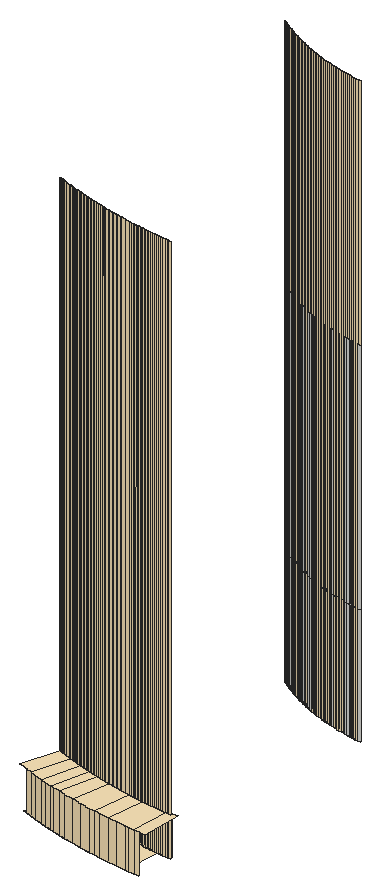
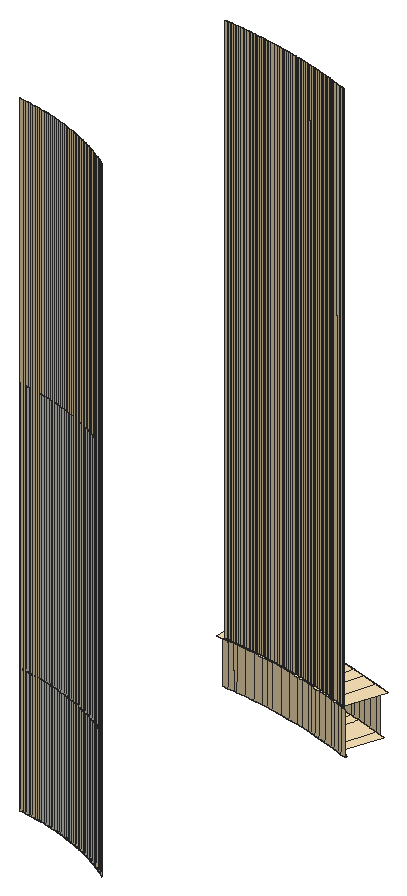
# SketchUp Ruby script. Lengths in inches.
U = 1.inch
M = Sketchup.active_model
def pt(a) = Geom::Point3d.new(a.map { |v| v * U })
def face(e, loops, mat)
  f = e.add_face(loops[0].map { |a| pt(a) })
  loops[1..].each { |l| e.add_face(l.map { |a| pt(a) }).erase! }
  f.material = f.back_material = mat if mat
  f
end
# faces: each face lists its corners as indices into pts; further lists are holes
def faces(e, pts, list, mat = nil) = list.each { |f| face(e, (f[0].is_a?(Array) ? f : [f]).map { |l| l.map { |i| pts[i] } }, mat) }
# xy, xz, yz: faces in a plane at the given z, y or x. An outline is a flat list of corners, or four numbers for a rectangle; further outlines are holes
def ring(l) = l.size == 4 ? [[l[0], l[1]], [l[2], l[1]], [l[2], l[3]], [l[0], l[3]]] : l.each_slice(2).to_a
def flat(e, list, mat, &to3) = list.each { |f| face(e, (f[0].is_a?(Array) ? f : [f]).map { |l| ring(l).map { |u, v| to3.(u, v) } }, mat) }
def xy(e, z, list, mat = nil) = flat(e, list, mat) { |x, y| [x, y, z] }
def xz(e, y, list, mat = nil) = flat(e, list, mat) { |x, z| [x, y, z] }
def yz(e, x, list, mat = nil) = flat(e, list, mat) { |y, z| [x, y, z] }
def lines(e, pts, list) = list.each { |a, b| e.add_line(pt(pts[a]), pt(pts[b])) }
# prism: a flat outline (further loops are holes) pulled along v
def prism(e, loops, v, mat = nil)
  f = face(e, loops, mat); d = Geom::Vector3d.new(v.map { |x| x * U })
  f.pushpull(f.normal.samedirection?(d) ? d.length : -d.length)
end
def box(e, o, s, mat = nil) = prism(e, [[o, [o[0] + s[0], o[1], o[2]], [o[0] + s[0], o[1] + s[1], o[2]], [o[0], o[1] + s[1], o[2]]]], [0, 0, s[2]], mat)
def at(x, y, z, deg = 0) = Geom::Transformation.translation(pt([x, y, z])) * Geom::Transformation.rotation(ORIGIN, Z_AXIS, deg.degrees)
def axes(o, x, y, z) = Geom::Transformation.new([*x, 0, *y, 0, *z, 0, *pt(o).to_a, 1])
def part(name) = M.definitions.add(name)
# library, detail: a bought-in or finely detailed component or shape, given as its bounding box
def library(name, o, s) = part(name).tap { |d| box(d.entities, o, s) }
def detail(e, o, s) = box(e.add_group.entities, o, s)
def put(e, d, t, mat = nil) = e.add_instance(d, t).tap { |i| i.material = mat if mat }
def group(e, t, mat = nil) = e.add_group.tap { |g| g.transformation = t; g.material = mat if mat }.entities
root = M.entities
M.materials.add("1026 AP 7946 SUNNY SIDE UP").color = [254, 231, 186]
xy(root,246,[[27.896,213.185,27.467,213.224,26.964,213.278,26.497,213.338,26.751,215.221,26.824,215.211,26.945,215.195,26.97,215.192,26.992,215.189,27.072,215.18,27.179,215.166,27.212,215.163,27.242,215.159,27.318,215.151,27.413,215.14,27.454,215.136,27.491,215.131,27.5625,215.124,27.648,215.116,27.697,215.111,27.741,215.107,27.806,215.101,27.882,215.094,27.94,215.089,27.992,215.084,28.05,215.08,28.055,215.079],[26.497,213.338,26.226,213.377,25.953,213.418,25.44,213.505,25.776,215.375,25.781,215.374,25.925,215.349,25.998,215.336,26.005,215.335,26.013,215.333,26.246,215.295,26.478,215.26,26.487,215.259,26.494,215.257,26.567,215.247,26.712,215.226,26.728,215.224,26.743,215.222,26.751,215.221],[25.44,213.505,24.926,213.603,24.465,213.699,24.87,215.555,24.94,215.54,25.01,215.524,25.047,215.517,25.087,215.508,25.181,215.489,25.256,215.473,25.286,215.468,25.318,215.461,25.424,215.441,25.503,215.425,25.525,215.421,25.549,215.416,25.67,215.394,25.75,215.379,25.765,215.377,25.776,215.375],[24.465,213.699,24.152,213.77,23.787,213.858,24.239,215.702,24.275,215.693,24.332,215.679,24.397,215.663,24.463,215.648,24.52,215.634,24.57,215.623,24.627,215.609,24.701,215.593,24.765,215.578,24.808,215.568,24.857,215.558,24.87,215.555],[23.787,213.858,23.573,213.912,23.274,213.99,23.768,215.823,23.788,215.818,23.857,215.8,23.94,215.778,23.988,215.765,24.031,215.754,24.095,215.738,24.168,215.719,24.225,215.705,24.239,215.702],
  [23.274,213.99,23.018,214.061,22.618,214.177,22.268,214.283,22.834,216.095,22.893,216.077,23.033,216.033,23.049,216.029,23.063,216.024,23.142,216.001,23.259,215.966,23.283,215.959,23.304,215.953,23.382,215.931,23.485,215.901,23.517,215.892,23.546,215.884,23.62,215.864,23.713,215.838,23.752,215.828,23.768,215.823],[22.268,214.283,22.016,214.364,21.774,214.444,22.379,216.242,22.584,216.175,22.808,216.103,22.816,216.101,22.823,216.098,22.834,216.095],[28.055,215.079,28.05,215.08,27.992,215.084,27.94,215.089,27.882,215.094,27.806,215.101,27.741,215.107,27.697,215.111,27.648,215.116,27.5625,215.124,27.491,215.131,27.454,215.136,27.413,215.14,27.318,215.151,27.242,215.159,27.212,215.163,27.179,215.166,27.072,215.18,26.992,215.189,26.97,215.192,26.945,215.195,26.824,215.211,26.751,215.221,26.764,215.32,27.198,215.265,27.664,215.214,28.064,215.178],[26.751,215.221,26.743,215.222,26.728,215.224,26.712,215.226,26.567,215.247,26.494,215.257,26.487,215.259,26.478,215.26,26.246,215.295,26.013,215.333,26.005,215.335,25.998,215.336,25.925,215.349,25.781,215.374,25.776,215.375,25.793,215.474,26.271,215.393,26.518,215.355,26.764,215.32],[25.776,215.375,25.765,215.377,25.75,215.379,25.67,215.394,25.549,215.416,25.525,215.421,25.503,215.425,25.424,215.441,25.318,215.461,25.286,215.468,25.256,215.473,25.181,215.489,25.087,215.508,25.047,215.517,25.01,215.524,24.94,215.54,24.87,215.555,24.891,215.653,25.317,215.564,25.793,215.474],
  [24.87,215.555,24.857,215.558,24.808,215.568,24.765,215.578,24.701,215.593,24.627,215.609,24.57,215.623,24.52,215.634,24.463,215.648,24.397,215.663,24.332,215.679,24.275,215.693,24.239,215.702,24.264,215.8,24.607,215.718,24.891,215.653],[24.239,215.702,24.225,215.705,24.168,215.719,24.095,215.738,24.031,215.754,23.988,215.765,23.94,215.778,23.857,215.8,23.788,215.818,23.768,215.823,23.794,215.922,24.072,215.848,24.264,215.8],[23.768,215.823,23.752,215.828,23.713,215.838,23.62,215.864,23.546,215.884,23.517,215.892,23.485,215.901,23.382,215.931,23.304,215.953,23.283,215.959,23.259,215.966,23.142,216.001,23.063,216.024,23.049,216.029,23.033,216.033,22.893,216.077,22.834,216.095,22.864,216.193,23.188,216.094,23.561,215.986,23.794,215.922],[22.834,216.095,22.823,216.098,22.816,216.101,22.808,216.103,22.584,216.175,22.379,216.242,22.411,216.34,22.634,216.266,22.864,216.193],[22.379,216.242,22.36,216.249,22.352,216.251,22.345,216.254,22.276,216.277,22.137,216.325,22.107,216.335,22.03,216.362,21.935,216.396,21.969,216.493,22.175,216.421,22.411,216.34]],"1026 AP 7946 SUNNY SIDE UP")
xy(root,248,[[28.983,213.12,29.064,215.118,28.752,215.132,28.503,215.147,28.378,213.151,28.649,213.135],[28.378,213.151,28.503,215.147,28.254,215.164,28.064,215.179,27.664,215.214,27.198,215.265,26.964,213.279,27.467,213.224,27.896,213.186,28.108,213.169],[26.964,213.279,27.198,215.265,26.765,215.32,26.518,215.355,26.226,213.377,26.497,213.338],[26.226,213.377,26.518,215.355,26.271,215.393,25.793,215.474,25.317,215.564,24.926,213.603,25.44,213.505,25.953,213.418],[24.926,213.603,25.317,215.564,24.891,215.653,24.607,215.718,24.152,213.77,24.465,213.699],
  [24.152,213.77,24.607,215.718,24.264,215.8,24.072,215.848,23.573,213.912,23.787,213.858],[23.573,213.912,24.072,215.848,23.794,215.922,23.561,215.986,23.018,214.061,23.274,213.99],[23.018,214.061,23.561,215.986,23.188,216.094,22.864,216.193,22.268,214.284,22.618,214.177],[22.268,214.284,22.864,216.193,22.634,216.266,22.412,216.34,22.175,216.421,21.519,214.531,21.774,214.444,22.016,214.364]],"1026 AP 7946 SUNNY SIDE UP")
p = [[28.649,213.135,246],[28.649,213.135,248],[28.378,213.151,248],[28.378,213.15,246],[27.467,213.224,246],[27.467,213.224,248],
  [26.964,213.279,248],[26.964,213.278,246],[27.896,213.185,246],[27.896,213.186,248],[28.108,213.169,246],[28.108,213.169,248],
  [26.497,213.338,246],[26.497,213.338,248],[26.226,213.377,248],[26.226,213.377,246],[25.953,213.418,246],[25.953,213.418,248],
  [25.44,213.505,248],[25.44,213.505,246],[24.926,213.603,248],[24.926,213.603,246],[24.465,213.699,248],[24.465,213.699,246],
  [24.152,213.77,248],[24.152,213.77,246],[23.787,213.858,248],[23.787,213.858,246],[23.573,213.912,246],[23.573,213.912,248],
  [23.274,213.99,248],[23.274,213.99,246],[23.018,214.061,248],[23.018,214.061,246],[22.618,214.177,248],[22.618,214.177,246],
  [22.268,214.284,248],[22.268,214.283,246],[22.016,214.364,248],[22.016,214.364,246],[28.428,215.052,246],[28.493,215.047,246],
  [28.493,215.047,274],[28.428,215.052,274],[28.538,215.045,246],[28.538,215.045,274],[28.587,215.042,246],[28.587,215.042,274],
  [28.673,215.037,246],[28.673,215.037,274],[28.744,215.033,246],[28.744,215.033,274],[27.318,215.151,246],[27.413,215.14,246],
  [27.413,215.14,274],[27.318,215.151,274],[27.454,215.136,246],[27.454,215.136,274],[27.491,215.131,246],[27.491,215.131,274],
  [27.5625,215.124,246],[27.5625,215.124,274],[27.648,215.116,246],[27.648,215.116,274],[27.697,215.111,246],[27.697,215.111,274],
  [27.741,215.107,246],[27.741,215.107,274],[27.806,215.101,246],[27.806,215.101,274],[27.882,215.094,246],[27.882,215.094,274],
  [27.94,215.089,246],[27.94,215.089,274],[27.992,215.084,246],[27.992,215.084,274],[28.05,215.08,246],[28.05,215.08,274],
  [28.055,215.079,246],[28.117,215.074,246],[28.117,215.074,274],[28.184,215.069,246],[28.184,215.069,274],[28.242,215.064,246],
  [28.242,215.064,274],[28.294,215.061,246],[28.294,215.061,274],[28.352,215.057,246],[28.352,215.057,274],[28.503,215.147,248],
  [28.503,215.146,246],[28.254,215.163,246],[28.254,215.164,248],[28.752,215.132,248],[28.752,215.132,246],[26.494,215.257,246],
  [26.567,215.247,246],[26.567,215.247,274],[26.494,215.257,274],[26.712,215.226,246],[26.712,215.226,274],[26.728,215.224,246],
  [26.728,215.224,274],[26.743,215.222,246],[26.743,215.222,274],[26.751,215.221,246],[26.824,215.211,246],[26.824,215.211,274],
  [26.945,215.195,246],[26.945,215.195,274],[26.97,215.192,246],[26.97,215.192,274],[26.992,215.189,246],[26.992,215.189,274],
  [27.072,215.18,246],[27.072,215.18,274],[27.179,215.166,246],[27.179,215.166,274],[27.212,215.163,246],[27.212,215.163,274],
  [27.242,215.159,246],[27.242,215.159,274],[27.664,215.214,248],[27.664,215.214,246],[27.198,215.265,246],[27.198,215.265,248],
  [28.064,215.179,248],[28.064,215.178,246],[25.781,215.374,246],[25.925,215.349,246],[25.925,215.349,274],[25.781,215.374,274],
  [25.998,215.336,246],[25.998,215.336,274],[26.005,215.335,246],[26.005,215.335,274],[26.013,215.333,246],[26.013,215.333,274],
  [26.246,215.295,246],[26.246,215.295,274],[26.478,215.26,246],[26.478,215.26,274],[26.487,215.259,246],[26.487,215.259,274],
  [26.765,215.32,248],[26.764,215.32,246],[26.518,215.355,246],[26.518,215.355,248],[25.318,215.461,246],[25.424,215.441,246],
  [25.424,215.441,274],[25.318,215.461,274],[25.503,215.425,246],[25.503,215.425,274],[25.525,215.421,246],[25.525,215.421,274],
  [25.549,215.416,246],[25.549,215.416,274],[25.67,215.394,246],[25.67,215.394,274],[25.75,215.379,246],[25.75,215.379,274],
  [25.765,215.377,246],[25.765,215.377,274],[25.776,215.375,246],[26.271,215.393,248],[26.271,215.393,246],[25.793,215.474,246],
  [25.793,215.474,248],[24.857,215.558,246],[24.87,215.555,246],[24.94,215.54,246],[24.94,215.54,274],[24.857,215.558,274],
  [25.01,215.524,246],[25.01,215.524,274],[25.047,215.517,246],[25.047,215.517,274],[25.087,215.508,246],[25.087,215.508,274],
  [25.181,215.489,246],[25.181,215.489,274],[25.256,215.473,246],[25.256,215.473,274],[25.286,215.468,246],[25.286,215.468,274],
  [25.317,215.564,246],[25.317,215.564,248],[24.397,215.663,246],[24.463,215.648,246],[24.463,215.648,274],[24.397,215.663,274],
  [24.52,215.634,246],[24.52,215.634,274],[24.57,215.623,246],[24.57,215.623,274],[24.627,215.609,246],[24.627,215.609,274],
  [24.701,215.593,246],[24.701,215.593,274],[24.765,215.578,246],[24.765,215.578,274],[24.808,215.568,246],[24.808,215.568,274],
  [24.891,215.653,246],[24.891,215.653,248],[24.031,215.754,246],[24.095,215.738,246],[24.095,215.738,274],[24.031,215.754,274],
  [24.168,215.719,246],[24.168,215.719,274],[24.225,215.705,246],[24.225,215.705,274],[24.239,215.702,246],[24.275,215.693,246],
  [24.275,215.693,274],[24.332,215.679,246],[24.332,215.679,274],[24.607,215.718,248],[24.607,215.718,246],[24.264,215.8,246],
  [24.264,215.8,248],[23.62,215.864,246],[23.713,215.838,246],[23.713,215.838,274],[23.62,215.864,274],[23.752,215.828,246],
  [23.752,215.828,274],[23.768,215.823,246],[23.788,215.818,246],[23.788,215.818,274],[23.857,215.8,246],[23.857,215.8,274],
  [24.072,215.848,248],[24.072,215.848,246],[23.794,215.922,246],[23.794,215.922,248],[23.94,215.778,246],[23.94,215.778,274],
  [23.988,215.765,246],[23.988,215.765,274],[23.304,215.953,246],[23.382,215.931,246],[23.382,215.931,274],[23.304,215.953,274],
  [23.485,215.901,246],[23.485,215.901,274],[23.517,215.892,246],[23.517,215.892,274],[23.546,215.884,246],[23.546,215.884,274],
  [23.561,215.986,246],[23.561,215.986,248],[22.893,216.077,246],[23.033,216.033,246],[23.033,216.033,274],[22.893,216.077,274],
  [23.049,216.029,246],[23.049,216.029,274],[23.063,216.024,246],[23.063,216.024,274],[23.142,216.001,246],[23.142,216.001,274],
  [23.259,215.966,246],[23.259,215.966,274],[23.188,216.094,246],[23.188,216.094,248],[23.283,215.959,246],[23.283,215.959,274],
  [22.584,216.175,246],[22.808,216.103,246],[22.808,216.103,274],[22.584,216.175,274],[22.816,216.101,246],[22.816,216.101,274],
  [22.823,216.098,246],[22.823,216.098,274],[22.834,216.095,246],[22.864,216.193,246],[22.864,216.193,248],[22.352,216.251,246],
  [22.36,216.249,246],[22.36,216.249,274],[22.352,216.251,274],[22.379,216.242,246],[22.634,216.266,246],[22.634,216.266,248],
  [22.107,216.335,246],[22.122,216.33,246],[22.122,216.33,274],[22.107,216.335,274],[22.137,216.325,246],[22.137,216.325,274],
  [22.276,216.277,246],[22.276,216.277,274],[22.412,216.34,248],[22.411,216.34,246],[22.175,216.421,246],[22.175,216.421,248],
  [22.345,216.254,246],[22.345,216.254,274],[21.969,216.493,246],[21.97,216.493,248],[28.123,227.148,252],[27.968,227.173,252],
  [27.968,227.173,246],[28.123,227.148,246],[28.123,227.148,246],[27.999,227.168,246],[27.999,227.168,276],[28.123,227.148,276],
  [28.278,227.124,252],[28.278,227.124,246],[28.247,227.129,246],[28.247,227.129,276],[28.371,227.111,246],[28.371,227.111,276],
  [28.434,227.103,252],[28.434,227.103,246],[28.59,227.083,252],[28.59,227.083,246],[28.496,227.095,246],[28.496,227.095,276],
  [28.621,227.08,246],[28.621,227.08,276],[28.746,227.066,252],[28.746,227.066,246],[28.746,227.066,246],[28.746,227.066,276],
  [27.659,227.231,252],[27.505,227.262,252],[27.505,227.262,246],[27.659,227.231,246],[27.628,227.237,246],[27.505,227.262,246],
  [27.505,227.262,276],[27.628,227.237,276],[27.751,227.213,246],[27.751,227.213,276],[27.813,227.201,252],[27.813,227.201,246],
  [27.875,227.19,246],[27.875,227.19,276],[27.199,227.332,252],[27.046,227.369,252],[27.046,227.369,246],[27.199,227.332,246],
  [27.138,227.346,246],[27.016,227.377,246],[27.016,227.377,276],[27.138,227.346,276],[27.26,227.317,246],[27.26,227.317,276],
  [27.352,227.296,252],[27.352,227.296,246],[27.382,227.289,246],[27.382,227.289,276],[26.894,227.409,252],[26.743,227.451,252],
  [26.743,227.451,246],[26.894,227.409,246],[26.773,227.442,246],[26.652,227.476,246],[26.652,227.476,276],[26.773,227.442,276],
  [26.894,227.409,246],[26.894,227.409,276],[26.442,227.54,252],[26.292,227.587,252],[26.292,227.587,246],[26.442,227.54,246],
  [26.412,227.549,246],[26.292,227.587,246],[26.292,227.587,276],[26.412,227.549,276],[26.592,227.494,252],[26.592,227.494,246],
  [26.532,227.512,246],[26.532,227.512,276],[26.143,227.637,252],[25.994,227.688,252],[25.994,227.688,246],[26.143,227.637,246],
  [26.172,227.627,246],[26.054,227.667,246],[26.054,227.667,276],[26.172,227.627,276],[25.847,227.742,252],[25.7,227.797,252],
  [25.7,227.797,246],[25.847,227.742,246],[25.935,227.709,246],[25.817,227.753,246],[25.817,227.753,276],[25.935,227.709,276],
  [25.583,227.843,246],[25.466,227.89,246],[25.466,227.89,276],[25.583,227.843,276],[25.553,227.854,252],[25.553,227.854,246],
  [25.7,227.797,246],[25.7,227.797,276],[25.35,227.9375,246],[25.234,227.987,246],[25.234,227.987,276],[25.35,227.9375,276],
  [25.408,227.913,252],[25.263,227.975,252],[25.263,227.975,246],[25.408,227.913,246],[25.119,228.037,252],[24.976,228.102,252],
  [24.976,228.102,246],[25.119,228.037,246],[25.119,228.037,246],[25.005,228.089,246],[25.005,228.089,276],[25.119,228.037,276],
  [24.834,228.169,252],[24.834,228.169,246],[24.891,228.142,246],[24.777,228.196,246],[24.777,228.196,276],[24.891,228.142,276],
  [24.693,228.238,252],[24.552,228.308,252],[24.552,228.308,246],[24.693,228.238,246],[24.664,228.251,246],[24.664,228.251,276],
  [24.413,228.38,252],[24.413,228.38,246],[24.552,228.308,246],[24.44,228.366,246],[24.44,228.366,276],[24.552,228.308,276],
  [24.329,228.424,246],[24.219,228.484,246],[24.219,228.484,276],[24.329,228.424,276],[24.274,228.454,252],[24.274,228.454,246],
  [24.137,228.53,252],[24,228.608,252],[24,228.608,246],[24.137,228.53,246],[24.109,228.545,246],[24,228.608,246],
  [24,228.608,276],[24.109,228.545,276],[23.864,228.687,252],[23.864,228.687,246],[23.892,228.671,246],[23.892,228.671,276],
  [23.73,228.768,252],[23.73,228.768,246],[23.784,228.736,246],[23.677,228.801,246],[23.677,228.801,276],[23.784,228.736,276],
  [23.597,228.851,252],[23.597,228.851,246],[23.57,228.868,246],[23.57,228.868,276],[23.464,228.936,252],[23.333,229.022,252],
  [23.333,229.022,246],[23.464,228.936,246],[23.464,228.936,246],[23.359,229.005,246],[23.359,229.005,276],[23.464,228.936,276],
  [28.123,227.148,264],[27.968,227.173,264],[27.968,227.173,252],[28.123,227.148,252],[28.278,227.124,264],[28.278,227.124,252],
  [28.434,227.103,264],[28.434,227.103,252],[28.59,227.083,264],[28.59,227.083,252],[28.746,227.066,264],[28.746,227.066,252],
  [27.659,227.231,264],[27.505,227.262,264],[27.505,227.262,252],[27.659,227.231,252],[27.813,227.201,264],[27.813,227.201,252],
  [27.199,227.332,264],[27.046,227.369,264],[27.046,227.369,252],[27.199,227.332,252],[27.352,227.296,264],[27.352,227.296,252],
  [26.894,227.409,264],[26.743,227.451,264],[26.743,227.451,252],[26.894,227.409,252],[26.442,227.54,264],[26.292,227.587,264],
  [26.292,227.587,252],[26.442,227.54,252],[26.592,227.494,264],[26.592,227.494,252],[26.143,227.637,264],[25.994,227.688,264],
  [25.994,227.688,252],[26.143,227.637,252],[25.847,227.742,264],[25.7,227.797,264],[25.7,227.797,252],[25.847,227.742,252],
  [25.553,227.854,264],[25.553,227.854,252],[25.408,227.913,264],[25.263,227.975,264],[25.263,227.975,252],[25.408,227.913,252],
  [25.119,228.037,264],[24.976,228.102,264],[24.976,228.102,252],[25.119,228.037,252],[24.834,228.169,264],[24.834,228.169,252],
  [24.693,228.238,264],[24.552,228.308,264],[24.552,228.308,252],[24.693,228.238,252],[24.413,228.38,264],[24.413,228.38,252],
  [24.274,228.454,264],[24.274,228.454,252],[24.137,228.53,264],[24,228.608,264],[24,228.608,252],[24.137,228.53,252],
  [23.864,228.687,264],[23.864,228.687,252],[23.73,228.768,264],[23.73,228.768,252],[23.597,228.851,264],[23.597,228.851,252],
  [23.464,228.936,264],[23.333,229.022,264],[23.333,229.022,252],[23.464,228.936,252]]
faces(root,p,[[0,1,2,3],[4,5,6,7],[8,9,5,4],[10,11,9,8],[3,2,11,10],[12,13,14,15],[7,6,13,12],[16,17,18,19],
  [15,14,17,16],[19,18,20,21],[21,20,22,23],[23,22,24,25],[25,24,26,27],[28,29,30,31],[27,26,29,28],[31,30,32,33],
  [33,32,34,35],[35,34,36,37],[37,36,38,39],[40,41,42,43],[41,44,45,42],[44,46,47,45],[46,48,49,47],[48,50,51,49],
  [52,53,54,55],[53,56,57,54],[56,58,59,57],[58,60,61,59],[60,62,63,61],[62,64,65,63],[64,66,67,65],[66,68,69,67],
  [68,70,71,69],[70,72,73,71],[72,74,75,73],[74,76,77,75],[76,78,79,80,77],[79,81,82,80],[81,83,84,82],[83,85,86,84],
  [85,87,88,86],[89,90,91,92],[87,40,43,88],[93,94,90,89],[95,96,97,98],[96,99,100,97],[99,101,102,100],[101,103,104,102],
  [103,105,106,107,104],[106,108,109,107],[108,110,111,109],[110,112,113,111],[112,114,115,113],[114,116,117,115],[116,118,119,117],[118,120,121,119],
  [120,52,55,121],[122,123,124,125],[126,127,123,122],[92,91,127,126],[128,129,130,131],[129,132,133,130],[132,134,135,133],[134,136,137,135],
  [136,138,139,137],[138,140,141,139],[140,142,143,141],[142,95,98,143],[144,145,146,147],[125,124,145,144],[148,149,150,151],[149,152,153,150],
  [152,154,155,153],[154,156,157,155],[156,158,159,157],[158,160,161,159],[160,162,163,161],[162,164,128,131,163],[165,166,167,168],[147,146,166,165],
  [169,170,171,172,173],[171,174,175,172],[174,176,177,175],[176,178,179,177],[178,180,181,179],[180,182,183,181],[182,184,185,183],[184,148,151,185],
  [168,167,186,187],[188,189,190,191],[189,192,193,190],[192,194,195,193],[194,196,197,195],[196,198,199,197],[198,200,201,199],[200,202,203,201],
  [202,169,173,203],[187,186,204,205],[206,207,208,209],[207,210,211,208],[210,212,213,211],[212,214,215,216,213],[215,217,218,216],[217,188,191,218],
  [219,220,221,222],[205,204,220,219],[223,224,225,226],[224,227,228,225],[227,229,230,231,228],[230,232,233,231],[234,235,236,237],[232,238,239,233],
  [238,240,241,239],[240,206,209,241],[222,221,235,234],[242,243,244,245],[243,246,247,244],[246,248,249,247],[248,250,251,249],[250,223,226,251],
  [237,236,252,253],[254,255,256,257],[255,258,259,256],[258,260,261,259],[260,262,263,261],[262,264,265,263],[253,252,266,267],[264,268,269,265],
  [268,242,245,269],[270,271,272,273],[271,274,275,272],[274,276,277,275],[276,278,254,257,277],[267,266,279,280],[281,282,283,284],[282,285,270,273,283],
  [280,279,286,287],[288,289,290,291],[289,292,293,290],[292,294,295,293],[296,297,298,299],[294,300,301,295],[300,281,284,301],[287,286,297,296],
  [299,298,302,303],[308,309,310,311],[314,308,311,315],[316,314,315,317],[322,316,317,323],[324,322,323,325],[328,324,325,329],[334,335,336,337],
  [338,334,337,339],[342,338,339,343],[309,342,343,310],[348,349,350,351],[352,348,351,353],[356,352,353,357],[335,356,357,336],[362,363,364,365],
  [366,362,365,367],[349,366,367,350],[372,373,374,375],[378,372,375,379],[363,378,379,364],[384,385,386,387],[373,384,387,374],[392,393,394,395],
  [385,392,395,386],[396,397,398,399],[402,396,399,403],[393,402,403,394],[404,405,406,407],[397,404,407,398],[416,417,418,419],[405,416,419,406],
  [422,423,424,425],[417,422,425,418],[423,430,431,424],[434,435,436,437],[430,434,437,431],[438,439,440,441],[435,438,441,436],[448,449,450,451],
  [439,448,451,440],[449,454,455,450],[458,459,460,461],[454,458,461,455],[459,464,465,460],[470,471,472,473],[464,470,473,465]],"1026 AP 7946 SUNNY SIDE UP")
faces(root,p,[[304,305,306,307],[312,304,307,313],[318,312,313,319],[320,318,319,321],[326,320,321,327],[330,331,332,333],[340,330,333,341],[305,340,341,306],
  [344,345,346,347],[354,344,347,355],[331,354,355,332],[358,359,360,361],[345,358,361,346],[368,369,370,371],[376,368,371,377],[359,376,377,360],
  [380,381,382,383],[369,380,383,370],[388,389,390,391],[381,388,391,382],[389,400,401,390],[408,409,410,411],[400,408,411,401],[412,413,414,415],
  [409,412,415,410],[413,420,421,414],[426,427,428,429],[420,426,429,421],[427,432,433,428],[432,442,443,433],[444,445,446,447],[442,444,447,443],
  [445,452,453,446],[452,456,457,453],[456,462,463,457],[466,467,468,469],[462,466,469,463],[474,475,476,477],[478,474,477,479],[480,478,479,481],
  [482,480,481,483],[484,482,483,485],[486,487,488,489],[490,486,489,491],[475,490,491,476],[492,493,494,495],[496,492,495,497],[487,496,497,488],
  [498,499,500,501],[493,498,501,494],[502,503,504,505],[506,502,505,507],[499,506,507,500],[508,509,510,511],[503,508,511,504],[512,513,514,515],
  [509,512,515,510],[513,516,517,514],[518,519,520,521],[516,518,521,517],[522,523,524,525],[519,522,525,520],[523,526,527,524],[528,529,530,531],
  [526,528,531,527],[529,532,533,530],[532,534,535,533],[536,537,538,539],[534,536,539,535],[537,540,541,538],[540,542,543,541],[542,544,545,543],
  [546,547,548,549],[544,546,549,545]])
